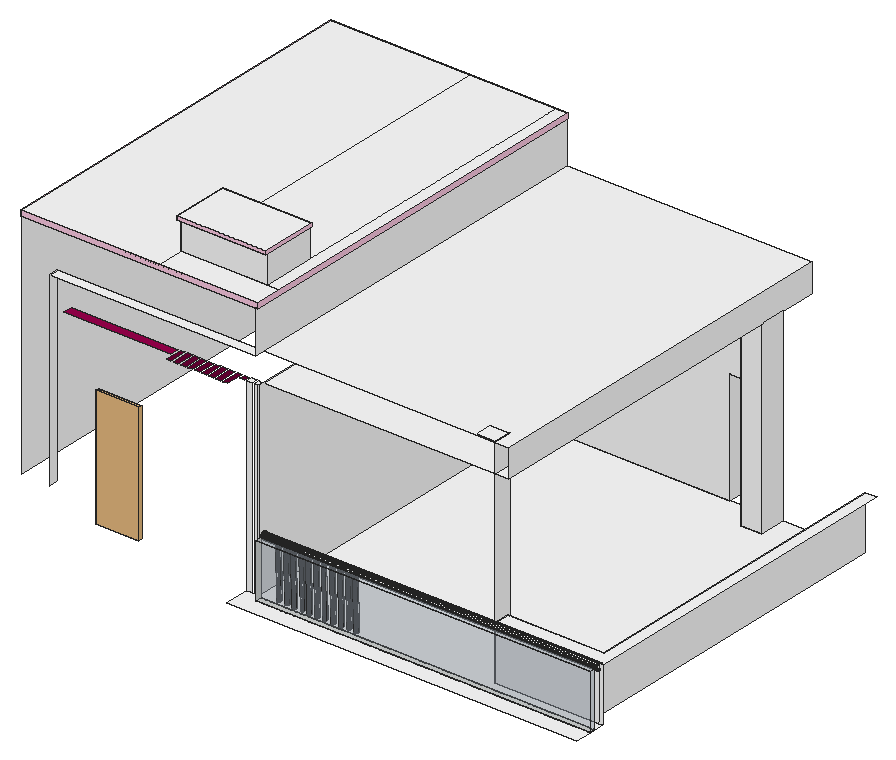
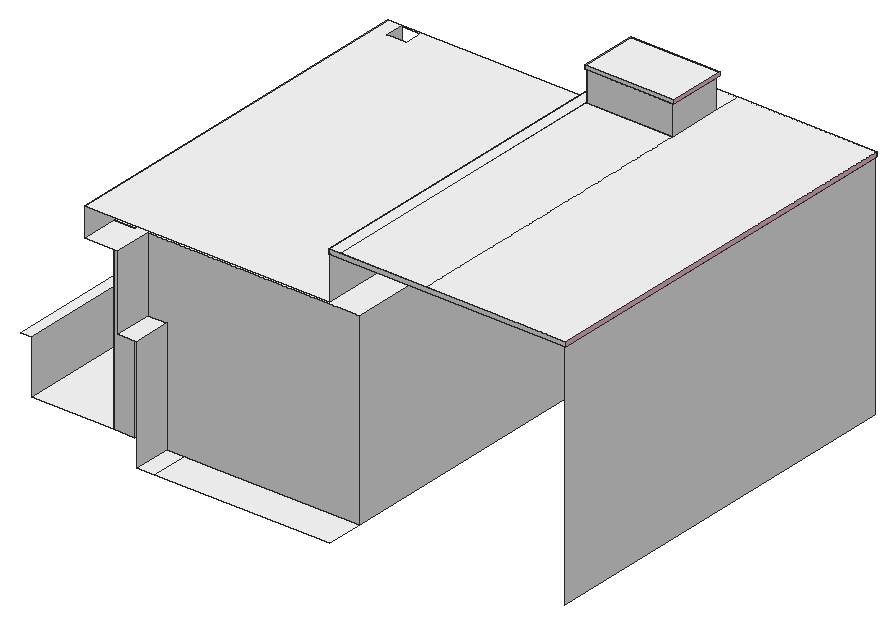
# SketchUp Ruby script. Lengths in inches.
U = 1.inch
M = Sketchup.active_model
def pt(a) = Geom::Point3d.new(a.map { |v| v * U })
def face(e, loops, mat)
  f = e.add_face(loops[0].map { |a| pt(a) })
  loops[1..].each { |l| e.add_face(l.map { |a| pt(a) }).erase! }
  f.material = f.back_material = mat if mat
  f
end
# faces: each face lists its corners as indices into pts; further lists are holes
def faces(e, pts, list, mat = nil) = list.each { |f| face(e, (f[0].is_a?(Array) ? f : [f]).map { |l| l.map { |i| pts[i] } }, mat) }
# xy, xz, yz: faces in a plane at the given z, y or x. An outline is a flat list of corners, or four numbers for a rectangle; further outlines are holes
def ring(l) = l.size == 4 ? [[l[0], l[1]], [l[2], l[1]], [l[2], l[3]], [l[0], l[3]]] : l.each_slice(2).to_a
def flat(e, list, mat, &to3) = list.each { |f| face(e, (f[0].is_a?(Array) ? f : [f]).map { |l| ring(l).map { |u, v| to3.(u, v) } }, mat) }
def xy(e, z, list, mat = nil) = flat(e, list, mat) { |x, y| [x, y, z] }
def xz(e, y, list, mat = nil) = flat(e, list, mat) { |x, z| [x, y, z] }
def yz(e, x, list, mat = nil) = flat(e, list, mat) { |y, z| [x, y, z] }
def lines(e, pts, list) = list.each { |a, b| e.add_line(pt(pts[a]), pt(pts[b])) }
# prism: a flat outline (further loops are holes) pulled along v
def prism(e, loops, v, mat = nil)
  f = face(e, loops, mat); d = Geom::Vector3d.new(v.map { |x| x * U })
  f.pushpull(f.normal.samedirection?(d) ? d.length : -d.length)
end
def box(e, o, s, mat = nil) = prism(e, [[o, [o[0] + s[0], o[1], o[2]], [o[0] + s[0], o[1] + s[1], o[2]], [o[0], o[1] + s[1], o[2]]]], [0, 0, s[2]], mat)
def at(x, y, z, deg = 0) = Geom::Transformation.translation(pt([x, y, z])) * Geom::Transformation.rotation(ORIGIN, Z_AXIS, deg.degrees)
def axes(o, x, y, z) = Geom::Transformation.new([*x, 0, *y, 0, *z, 0, *pt(o).to_a, 1])
def part(name) = M.definitions.add(name)
# library, detail: a bought-in or finely detailed component or shape, given as its bounding box
def library(name, o, s) = part(name).tap { |d| box(d.entities, o, s) }
def detail(e, o, s) = box(e.add_group.entities, o, s)
def put(e, d, t, mat = nil) = e.add_instance(d, t).tap { |i| i.material = mat if mat }
def group(e, t, mat = nil) = e.add_group.tap { |g| g.transformation = t; g.material = mat if mat }.entities
root = M.entities
M.materials.add("Glass_Basic_01").color = [161, 173, 186]
M.materials["Glass_Basic_01"].alpha = 0.25
M.materials.add("L01_Cotton_Candy").color = [255, 204, 229]
M.materials.add("L07_Raspberry_Rush").color = [153, 0, 76]
M.materials.add("L08_Velvet_Rose").color = [102, 0, 51]
M.materials.add("M00_Soft_Cloud").color = [255, 255, 255]
c1 = library("Window 109 023",[-16.24,-1.39,-0.03],[32.48,2.78,89.27])
xy(root,396,[[202.46,150.61,484.6,155.72]])
xy(root,396,[[189,136.44,484.6,136.44,484.6,150.61,202.46,150.61,202.46,155.72,484.6,155.72,484.6,163.42,394.03,163.42,394.03,176.81,475.23,176.81,475.23,451.98,405.98,451.98,405.98,429.82,388.44,429.82,388.44,451.29,199,451.29,199,158.82,198,158.82,198,158.3,189,158.3],[388.44,429.82,405.98,451.98],[199,451.29,346.72,482.39],[346.72,451.29,361.66,482.39]],"M00_Soft_Cloud")
xy(root,437.32,[[198.42,161.79,483.26,161.82]],"M00_Soft_Cloud")
xy(root,441.51,[[394.03,163.42,481.66,164.21],[481.66,163.42,484.6,163.42,484.6,451.98,475.23,451.98,475.23,176.81,394.03,176.81,394.03,164.21,481.66,164.21]],"M00_Soft_Cloud")
xy(root,441.75,[[202.46,150.61,484.6,155.72]],"Glass_Basic_01")
xy(root,491.38,[[361.66,451.29,377.86,482.39]],"M00_Soft_Cloud")
xy(root,554.29,[[37,154.91,127,162.91]],"L07_Raspberry_Rush")
xy(root,554.29,[[129,148,133,162.91],[135,148,139,162.91],[141,148,145,162.91],[147,148,151,162.91],[153,148,157,162.91],
  [159,148,163,162.91],[165,148,169,162.91],[171,148,175,162.91],[177,148,181,162.91],[183,158.3,187,162.91]],"L08_Velvet_Rose")
xy(root,554.29,[[189,158.3,193,162.91],[195,158.3,198,162.91],[198,158.82,199,162.91],[199,162.91,199,451.29,377.86,451.29,377.86,420,405.98,420,405.98,162.91],[377.86,420,377.86,482.39,405.98,482.39,405.98,451.98,388.44,451.98,388.44,429.82,405.98,429.82,405.98,420],
  [388.44,429.82,405.98,451.98]],"M00_Soft_Cloud")
xy(root,578.29,[[25,155.3,199,162.91],[[199,162.91,405.98,482.39],[377.49,163.42,394.03,178.61]]],"M00_Soft_Cloud")
xy(root,614.29,[[0,155.3,1,158.3],[1,155.3,199,482.39],[199,155.3,200,158.3],[0,158.3,1,482.39],[199,158.3,200,482.39]],"M00_Soft_Cloud")
xy(root,618.29,[[0,155.3,117.07,482.39],[117.07,155.3,200,178.22],[117.07,178.22,190.22,223.17],[190.22,178.22,200,482.39],[117.07,223.17,190.22,482.39]],"M00_Soft_Cloud")
xy(root,643.14,[[116.07,175.22,191.22,178.22],[116.07,178.22,117.07,223.17],[190.22,178.22,191.22,223.17]],"L01_Cotton_Candy")
xy(root,643.14,[[117.07,178.22,190.22,223.17]],"M00_Soft_Cloud")
xy(root,646.14,[[116.07,175.22,191.22,223.17]],"M00_Soft_Cloud")
xz(root,150.61,[[202.46,396,484.6,441.75]],"Glass_Basic_01")
xz(root,155.3,[[0,614.29,200,618.29]],"L01_Cotton_Candy")
xz(root,155.72,[[202.46,396,484.6,441.75]],"Glass_Basic_01")
xz(root,158.3,[[189,396,193,554.29],[195,396,198,554.29]],"M00_Soft_Cloud")
xz(root,158.82,[[198,396,199,554.29]],"M00_Soft_Cloud")
xz(root,163.42,[[394.03,396,481.66,441.51],[481.66,396,484.6,441.51]],"M00_Soft_Cloud")
xz(root,175.22,[[116.07,643.14,191.22,646.14]],"L01_Cotton_Candy")
xz(root,176.81,[[394.03,396,398.01,441.51],[398.01,396,475.23,441.51]],"M00_Soft_Cloud")
xz(root,178.22,[[117.07,618.29,190.22,643.14]],"M00_Soft_Cloud")
xz(root,223.17,[[117.07,618.29,190.22,643.14],[116.07,643.14,191.22,646.14]],"M00_Soft_Cloud")
xz(root,429.82,[[388.44,396,405.98,554.29]],"M00_Soft_Cloud")
xz(root,451.29,[[199,396,361.66,396,361.66,491.38,377.86,491.38,377.86,554.29,199,554.29]],"M00_Soft_Cloud")
xz(root,451.98,[[388.44,396,405.98,554.29]],"M00_Soft_Cloud")
xz(root,482.39,[[0,614.29,200,618.29]],"M00_Soft_Cloud")
yz(root,0,[[155.3,614.29,482.39,618.29]],"L01_Cotton_Candy")
yz(root,1,[[155.3,419.15,482.39,614.29]],"M00_Soft_Cloud")
yz(root,25,[[155.3,419.15,162.91,578.29]],"M00_Soft_Cloud")
yz(root,116.07,[[175.22,643.14,223.17,646.14]],"L01_Cotton_Candy")
yz(root,117.07,[[178.22,618.29,223.17,643.14]],"M00_Soft_Cloud")
yz(root,190.22,[[178.22,618.29,223.17,643.14]],"M00_Soft_Cloud")
yz(root,191.22,[[175.22,643.14,223.17,646.14]],"L01_Cotton_Candy")
yz(root,198,[[158.3,396,158.82,554.29]],"M00_Soft_Cloud")
yz(root,199,[[158.82,396,451.29,554.29],[155.3,578.29,482.39,614.29]],"M00_Soft_Cloud")
yz(root,200,[[155.3,614.29,482.39,618.29]],"L01_Cotton_Candy")
yz(root,202.46,[[150.61,396,155.72,441.75]])
yz(root,361.66,[[451.29,396,482.39,491.38]],"M00_Soft_Cloud")
yz(root,377.86,[[451.29,491.38,482.39,554.29]],"M00_Soft_Cloud")
yz(root,388.44,[[429.82,396,451.98,554.29]],"M00_Soft_Cloud")
yz(root,394.03,[[163.42,396,176.81,441.51],[176.81,396,178.61,396,178.61,578.29,163.42,578.29,163.42,441.51,176.81,441.51]],"M00_Soft_Cloud")
yz(root,405.98,[[429.82,396,451.98,554.29],[162.91,554.29,482.39,578.29]],"M00_Soft_Cloud")
yz(root,475.23,[[176.81,396,451.98,441.51]],"M00_Soft_Cloud")
yz(root,484.6,[[150.61,396,155.72,441.75]],"Glass_Basic_01")
p = [[253.49,156.28,440.79],[253.49,157.49,396],[253.91,157.4375,396],[253.91,156.23,440.79],[254.32,157.49,396],[254.32,156.28,440.79],
  [246.48,156.5,440.8],[246.48,157.7,396],[246.87,157.54,396],[246.87,156.34,440.79],[247.28,157.49,396],[247.28,156.28,440.79],
  [247.69,157.54,396],[247.69,156.34,440.79],[248.08,157.7,396],[248.08,156.5,440.8],[253.11,156.44,440.8],[253.11,157.65,396],
  [254.7,157.65,396],[254.7,156.44,440.8],[227.77,156.48,440.79],[227.77,157.6875,396],[228.18,157.63,396],[228.18,156.42,440.79],
  [228.6,157.6875,396],[228.6,156.48,440.79],[252.78,156.69,440.8],[252.78,157.9,396],[255.04,157.9,396],[255.04,156.69,440.8],
  [260.23,156.48,440.79],[260.23,157.68,396],[260.65,157.63,396],[260.65,156.42,440.79],[261.06,157.68,396],[261.06,156.48,440.79],
  [227.38,156.64,440.8],[227.38,157.85,396],[228.98,157.85,396],[228.98,156.64,440.8],[246.15,156.75,440.8],[246.15,157.96,396],
  [248.41,157.96,396],[248.41,156.75,440.8],[259.85,156.64,440.8],[259.85,157.84,396],[261.44,157.84,396],[261.44,156.64,440.8],
  [267.02,156.68,440.8],[267.02,157.89,396],[267.4,157.73,396],[267.4,156.52,440.79],[267.82,157.68,396],[267.82,156.47,440.79],
  [268.23,157.73,396],[268.23,156.52,440.79],[268.62,157.89,396],[268.62,156.68,440.8],[227.05,156.89,440.8],[227.05,158.1,396],
  [229.3125,158.1,396],[229.3125,156.89,440.8],[259.52,156.89,440.8],[259.52,158.1,396],[261.78,158.1,396],[261.78,156.89,440.8],
  [245.9,157.08,440.8125],[245.9,158.29,396],[248.66,158.29,396],[248.66,157.08,440.8125],[252.52,157.03,440.8125],[252.52,158.23,396],
  [255.29,158.23,396],[255.29,157.03,440.8125],[266.6875,156.94,440.8],[266.6875,158.14,396],[268.95,158.14,396],[268.95,156.94,440.8],
  [279.15,156.99,440.8],[279.15,158.2,396],[279.53,158.04,396],[279.53,156.83,440.79],[279.95,157.99,396],[279.95,156.78,440.79],
  [280.36,158.04,396],[280.36,156.83,440.79],[280.74,158.2,396],[280.74,156.99,440.8],[226.8,157.22,440.8125],[226.8,158.43,396],
  [229.57,158.43,396],[229.57,157.22,440.8125],[239.74,157.07,440.8],[239.74,158.28,396],[240.125,158.12,396],[240.125,156.91,440.79],
  [240.54,158.0625,396],[240.54,156.85,440.79],[240.95,158.12,396],[240.95,156.91,440.79],[241.34,158.28,396],[241.34,157.07,440.8],
  [259.26,157.22,440.8125],[259.26,158.43,396],[262.03,158.43,396],[262.03,157.22,440.8125],[266.43,157.27,440.8125],[266.43,158.48,396],
  [269.2,158.48,396],[269.2,157.27,440.8125],[252.36,157.41,440.82],[252.36,158.62,396],[255.45,158.62,396],[255.45,157.41,440.82],
  [278.82,157.24,440.8],[278.82,158.45,396],[281.08,158.45,396],[281.08,157.24,440.8],[239.41,157.32,440.8],[239.41,158.53,396],
  [241.67,158.53,396],[241.67,157.32,440.8],[245.74,157.47,440.82],[245.74,158.67,396],[248.82,158.67,396],[248.82,157.47,440.82],
  [226.64,157.61,440.82],[226.64,158.82,396],[229.73,158.82,396],[229.73,157.61,440.82],[259.1,157.61,440.82],[259.1,158.81,396],
  [262.1875,158.81,396],[262.1875,157.61,440.82],[278.5625,157.58,440.8125],[278.5625,158.78,396],[281.33,158.78,396],[281.33,157.58,440.8125],
  [234,157.37,440.79],[234,158.58,396],[234.42,158.53,396],[234.42,157.32,440.79],[234.83,158.58,396],[234.83,157.37,440.79],
  [239.15,157.65,440.8125],[239.15,158.86,396],[241.92,158.86,396],[241.92,157.65,440.8125],[266.27,157.65,440.82],[266.27,158.86,396],
  [269.36,158.86,396],[269.36,157.65,440.82],[233.62,157.53,440.8],[233.62,158.74,396],[235.21,158.74,396],[235.21,157.53,440.8],
  [252.31,157.82,440.83],[252.31,159.03,396],[255.5,159.03,396],[255.5,157.82,440.83],[272.5625,157.59,440.8],[272.5625,158.8,396],
  [272.95,158.64,396],[272.95,157.43,440.79],[273.36,158.59,396],[273.36,157.38,440.79],[273.77,158.64,396],[273.77,157.43,440.79],
  [274.16,158.8,396],[274.16,157.59,440.8],[233.29,157.78,440.8],[233.29,158.99,396],[235.55,158.99,396],[235.55,157.78,440.8],
  [245.68,157.88,440.83],[245.68,159.09,396],[248.88,159.09,396],[248.88,157.88,440.83],[213.7,157.7,440.79],[213.7,158.91,396],
  [214.11,158.86,396],[214.11,157.65,440.79],[214.52,158.91,396],[214.52,157.7,440.79],[226.58,158.02,440.83],[226.58,159.23,396],
  [229.78,159.23,396],[229.78,158.02,440.83],[259.05,158.02,440.83],[259.05,159.23,396],[262.24,159.23,396],[262.24,158.02,440.83],
  [272.23,157.85,440.8],[272.23,159.06,396],[274.49,159.06,396],[274.49,157.85,440.8],[278.4,157.96,440.82],[278.4,159.17,396],
  [281.49,159.17,396],[281.49,157.96,440.82],[213.3125,157.86,440.8],[213.3125,159.07,396],[214.91,159.07,396],[214.91,157.86,440.8],
  [220.625,157.78,440.79],[220.625,158.99,396],[221.04,158.9375,396],[221.04,157.73,440.79],[221.45,158.99,396],[221.45,157.78,440.79],
  [238.99,158.04,440.82],[238.99,159.25,396],[242.08,159.25,396],[242.08,158.04,440.82],[266.22,158.06,440.83],[266.22,159.27,396],
  [269.41,159.27,396],[269.41,158.06,440.83],[220.24,157.94,440.8],[220.24,159.15,396],[221.84,159.15,396],[221.84,157.94,440.8],
  [233.03,158.12,440.8125],[233.03,159.32,396],[235.8,159.32,396],[235.8,158.12,440.8125],[252.36,159.45,396.01],[252.36,158.24,440.84],
  [255.45,159.45,396.01],[255.45,158.24,440.84],[271.98,158.18,440.8125],[271.98,159.39,396],[274.74,159.39,396],[274.74,158.18,440.8125],
  [212.98,158.11,440.8],[212.98,159.32,396],[215.24,159.32,396],[215.24,158.11,440.8],[219.91,158.2,440.8],[219.91,159.4,396],
  [222.17,159.4,396],[222.17,158.2,440.8],[245.74,159.5,396.01],[245.74,158.29,440.84],[248.82,159.5,396.01],[248.82,158.29,440.84],
  [226.64,159.64,396.01],[226.64,158.43,440.84],[229.73,159.64,396.01],[229.73,158.43,440.84],[238.94,158.45,440.83],[238.94,159.66,396],
  [242.14,159.66,396],[242.14,158.45,440.83],[259.1,159.64,396.01],[259.1,158.43,440.84],[262.1875,159.64,396.01],[262.1875,158.43,440.84],
  [278.35,158.375,440.83],[278.35,159.58,396],[281.54,159.58,396],[281.54,158.375,440.83],[212.73,158.45,440.8125],[212.73,159.65,396],
  [215.49,159.65,396],[215.49,158.45,440.8125],[232.87,158.5,440.82],[232.87,159.71,396],[235.96,159.71,396],[235.96,158.5,440.82],
  [266.27,159.6875,396.01],[266.27,158.48,440.84],[269.36,159.6875,396.01],[269.36,158.48,440.84],[219.65,158.53,440.8125],[219.65,159.74,396],
  [222.42,159.74,396],[222.42,158.53,440.8125],[252.52,159.83,396.02],[252.52,158.62,440.85],[255.29,159.83,396.02],[255.29,158.62,440.85],
  [271.82,158.5625,440.82],[271.82,159.77,396],[274.9,159.77,396],[274.9,158.5625,440.82],[245.9,159.89,396.02],[245.9,158.68,440.85],
  [248.66,159.89,396.02],[248.66,158.68,440.85],[212.57,158.83,440.82],[212.57,160.04,396],[215.65,160.04,396],[215.65,158.83,440.82],
  [226.8,160.03,396.02],[226.8,158.82,440.85],[229.57,160.03,396.02],[229.57,158.82,440.85],[259.26,160.03,396.02],[259.26,158.82,440.85],
  [262.03,160.03,396.02],[262.03,158.82,440.85],[278.4,160,396.01],[278.4,158.79,440.84],[281.49,160,396.01],[281.49,158.79,440.84],
  [219.49,158.91,440.82],[219.49,160.12,396],[222.58,160.12,396],[222.58,158.91,440.82],[232.82,158.91,440.83],[232.82,160.125,396],
  [236.01,160.125,396],[236.01,158.91,440.83],[238.99,160.07,396.01],[238.99,158.86,440.84],[242.08,160.07,396.01],[242.08,158.86,440.84],
  [266.43,160.07,396.02],[266.43,158.86,440.85],[269.2,160.07,396.02],[269.2,158.86,440.85],[252.78,160.16,396.03],[252.78,158.95,440.86],
  [255.04,160.16,396.03],[255.04,158.95,440.86],[271.76,158.98,440.83],[271.76,160.1875,396],[274.96,160.1875,396],[274.96,158.98,440.83],
  [246.15,160.22,396.03],[246.15,159.01,440.86],[248.41,160.22,396.03],[248.41,159.01,440.86],[212.51,159.24,440.83],[212.51,160.45,396],
  [215.71,160.45,396],[215.71,159.24,440.83],[227.05,160.36,396.03],[227.05,159.15,440.86],[229.3125,160.36,396.03],[229.3125,159.15,440.86],
  [259.52,160.36,396.03],[259.52,159.15,440.86],[261.78,160.36,396.03],[261.78,159.15,440.86],[278.5625,160.38,396.02],[278.5625,159.17,440.85],
  [281.33,160.38,396.02],[281.33,159.17,440.85],[219.44,159.32,440.83],[219.44,160.53,396],[222.64,160.53,396],[222.64,159.32,440.83],
  [232.87,160.54,396.01],[232.84,159.1,440.84],[232.87,159.33,440.84],[235.96,160.54,396.01],[235.96,159.33,440.84],[235.99,159.1,440.84],
  [239.15,160.46,396.02],[239.15,159.25,440.85],[241.92,160.46,396.02],[241.92,159.25,440.85],[266.6875,160.4,396.03],[266.6875,159.19,440.86],
  [268.95,160.4,396.03],[268.95,159.19,440.86],[246.48,160.47,396.04],[246.48,159.26,440.87],[248.08,160.47,396.04],[248.08,159.26,440.87],
  [253.11,160.42,396.04],[253.11,159.21,440.87],[254.7,160.42,396.04],[254.7,159.21,440.87],[271.82,160.6,396.01],[271.82,159.39,440.84],
  [274.9,160.6,396.01],[274.9,159.39,440.84],[259.85,160.61,396.04],[259.85,159.4,440.87],[261.44,160.61,396.04],[261.44,159.4,440.87],
  [212.57,160.87,396.01],[212.57,159.66,440.84],[215.65,160.87,396.01],[215.65,159.66,440.84],[227.38,160.61,396.04],[227.38,159.4,440.87],
  [228.98,160.61,396.04],[228.98,159.4,440.87],[239.41,160.79,396.03],[239.41,159.58,440.86],[241.67,160.79,396.03],[241.67,159.58,440.86],
  [253.49,160.58,396.04],[253.49,159.37,440.875],[254.32,160.58,396.04],[254.32,159.37,440.875],[267.02,160.66,396.04],[267.02,159.45,440.87],
  [268.62,160.66,396.04],[268.62,159.45,440.87],[278.82,160.71,396.03],[278.82,159.5,440.86],[281.08,160.71,396.03],[281.08,159.5,440.86],
  [219.49,160.95,396.01],[219.49,159.74,440.84],[222.58,160.95,396.01],[222.58,159.74,440.84],[233.03,160.92,396.02],[233.03,159.71,440.85],
  [235.8,160.92,396.02],[235.8,159.71,440.85],[246.87,160.63,396.04],[246.87,159.42,440.875],[247.69,160.63,396.04],[247.69,159.42,440.875],
  [227.77,160.77,396.04],[227.77,159.5625,440.875],[228.6,160.77,396.04],[228.6,159.5625,440.875],[247.28,160.69,396.04],[247.28,159.48,440.875],
  [253.91,160.63,396.04],[253.91,159.42,440.875],[260.23,160.77,396.04],[260.23,159.5625,440.875],[261.06,160.77,396.04],[261.06,159.5625,440.875],
  [267.4,160.82,396.04],[267.4,159.61,440.875],[268.23,160.82,396.04],[268.23,159.61,440.875],[271.98,160.99,396.02],[271.98,159.78,440.85],
  [274.74,160.99,396.02],[274.74,159.78,440.85],[279.15,160.97,396.04],[279.15,159.76,440.87],[280.74,160.97,396.04],[280.74,159.76,440.87],
  [228.18,160.83,396.04],[228.18,159.62,440.875],[239.74,161.04,396.04],[239.74,159.83,440.87],[241.34,161.04,396.04],[241.34,159.83,440.87],
  [260.65,160.83,396.04],[260.65,159.62,440.875],[267.82,160.87,396.04],[267.82,159.66,440.875],[212.73,161.25,396.02],[212.73,160.04,440.85],
  [215.49,161.25,396.02],[215.49,160.04,440.85],[219.65,161.33,396.02],[219.65,160.125,440.85],[222.42,161.33,396.02],[222.42,160.125,440.85],
  [233.29,161.25,396.03],[233.29,160.04,440.86],[235.55,161.25,396.03],[235.55,160.04,440.86],[240.125,161.2,396.04],[240.125,159.99,440.875],
  [240.95,161.2,396.04],[240.95,159.99,440.875],[272.23,161.32,396.03],[272.23,160.11,440.86],[274.49,161.32,396.03],[274.49,160.11,440.86],
  [279.53,161.125,396.04],[279.53,159.92,440.875],[280.36,161.125,396.04],[280.36,159.92,440.875],[279.95,161.18,396.04],[279.95,159.97,440.875],
  [212.98,161.58,396.03],[212.98,160.37,440.86],[215.24,161.58,396.03],[215.24,160.37,440.86],[233.62,161.51,396.04],[233.62,160.3,440.87],
  [235.21,161.51,396.04],[235.21,160.3,440.87],[240.54,161.26,396.04],[240.54,160.05,440.875],[219.91,161.66,396.03],[219.91,160.45,440.86],
  [222.17,161.66,396.03],[222.17,160.45,440.86],[272.5625,161.57,396.04],[272.5625,160.36,440.87],[274.16,161.57,396.04],[274.16,160.36,440.87],
  [234,161.67,396.04],[234,160.46,440.875],[234.83,161.67,396.04],[234.83,160.46,440.875],[213.3125,161.84,396.04],[213.3125,160.625,440.87],
  [214.91,161.84,396.04],[214.91,160.625,440.87],[272.95,161.73,396.04],[272.95,160.52,440.875],[273.77,161.73,396.04],[273.77,160.52,440.875],
  [220.24,161.92,396.04],[220.24,160.71,440.87],[221.84,161.92,396.04],[221.84,160.71,440.87],[234.42,161.72,396.04],[234.42,160.51,440.875],
  [273.36,161.78,396.04],[273.36,160.57,440.875],[213.7,162,396.04],[213.7,160.79,440.875],[214.52,162,396.04],[214.52,160.79,440.875],
  [220.625,162.08,396.04],[220.625,160.87,440.875],[221.45,162.08,396.04],[221.45,160.87,440.875],[214.11,162.05,396.04],[214.11,160.84,440.875],
  [221.04,162.13,396.04],[221.04,160.92,440.875],[483.26,161.07,437.42],[198.42,161.07,437.42],[198.42,161.79,437.32],[483.26,161.79,437.32],
  [214.37,161.82,437.32],[211.17,161.82,437.32],[198.42,161.82,437.32],[198.42,162.52,437.42],[483.26,162.52,437.42],[483.26,161.82,437.32],
  [269.19,161.82,437.32],[265.99,161.82,437.32],[261.87,161.82,437.32],[258.67,161.82,437.32],[254.93,161.82,437.32],[251.74,161.82,437.32],
  [248.04,161.82,437.32],[244.84,161.82,437.32],[241.38,161.82,437.32],[238.1875,161.82,437.32],[235.53,161.82,437.32],[232.34,161.82,437.32],
  [228.79,161.82,437.32],[225.6,161.82,437.32],[221.49,161.82,437.32],[218.29,161.82,437.32],[483.26,160.4,437.69],[198.42,160.4,437.69],
  [198.42,163.19,437.69],[483.26,163.19,437.69],[483.26,159.82,438.14],[198.42,159.82,438.14],[198.42,163.77,438.14],[483.26,163.77,438.14],
  [483.26,159.375,438.72],[198.42,159.375,438.72],[198.42,164.21,438.72],[483.26,164.21,438.72],[483.26,159.1,439.39],[198.42,159.1,439.39],
  [198.42,164.49,439.39],[483.26,164.49,439.39],[483.26,159,440.11],[198.42,159,440.11],[198.42,164.59,440.11],[483.26,164.59,440.11],
  [198.42,159.1,440.84],[483.26,159.1,440.84],[198.42,164.49,440.84],[483.26,164.49,440.84],[483.26,159.375,441.51],[198.42,159.375,441.51],
  [198.42,164.21,441.51],[394.03,164.21,441.51],[481.66,164.21,441.51],[483.26,164.21,441.51],[483.26,159.82,442.09],[198.42,159.82,442.09],
  [198.42,163.77,442.09],[483.26,163.77,442.09],[483.26,160.4,442.53],[198.42,160.4,442.53],[198.42,163.19,442.53],[483.26,163.19,442.53],
  [483.26,161.07,442.8125],[198.42,161.07,442.8125],[198.42,162.52,442.8125],[483.26,162.52,442.8125],[483.26,161.79,442.91],[198.42,161.79,442.91]]
faces(root,p,[[0,1,2,3],[3,2,4,5],[6,7,8,9],[9,8,10,11],[11,10,12,13],[13,12,14,15],[16,17,1,0],[5,4,18,19],
  [20,21,22,23],[23,22,24,25],[26,27,17,16],[19,18,28,29],[30,31,32,33],[33,32,34,35],[36,37,21,20],[25,24,38,39],
  [40,41,7,6],[15,14,42,43],[44,45,31,30],[35,34,46,47],[48,49,50,51],[51,50,52,53],[53,52,54,55],[55,54,56,57],
  [58,59,37,36],[39,38,60,61],[62,63,45,44],[47,46,64,65],[66,67,41,40],[43,42,68,69],[70,71,27,26],[29,28,72,73],
  [74,75,49,48],[57,56,76,77],[78,79,80,81],[81,80,82,83],[83,82,84,85],[85,84,86,87],[88,89,59,58],[61,60,90,91],
  [92,93,94,95],[95,94,96,97],[97,96,98,99],[99,98,100,101],[102,103,63,62],[65,64,104,105],[106,107,75,74],[77,76,108,109],
  [110,111,71,70],[73,72,112,113],[114,115,79,78],[87,86,116,117],[118,119,93,92],[101,100,120,121],[122,123,67,66],[69,68,124,125],
  [126,127,89,88],[91,90,128,129],[130,131,103,102],[105,104,132,133],[134,135,115,114],[117,116,136,137],[138,139,140,141],[141,140,142,143],
  [144,145,119,118],[121,120,146,147],[148,149,107,106],[109,108,150,151],[152,153,139,138],[143,142,154,155],[156,157,111,110],[113,112,158,159],
  [160,161,162,163],[163,162,164,165],[165,164,166,167],[167,166,168,169],[170,171,153,152],[155,154,172,173],[174,175,123,122],[125,124,176,177],
  [178,179,180,181],[181,180,182,183],[184,185,127,126],[129,128,186,187],[188,189,131,130],[133,132,190,191],[192,193,161,160],[169,168,194,195],
  [196,197,135,134],[137,136,198,199],[200,201,179,178],[183,182,202,203],[204,205,206,207],[207,206,208,209],[210,211,145,144],[147,146,212,213],
  [214,215,149,148],[151,150,216,217],[218,219,205,204],[209,208,220,221],[222,223,171,170],[173,172,224,225],[226,157,156,227],[158,228,229,159],
  [230,231,193,192],[195,194,232,233],[234,235,201,200],[203,202,236,237],[238,239,219,218],[221,220,240,241],[242,175,174,243],[176,244,245,177],
  [246,185,184,247],[186,248,249,187],[250,251,211,210],[213,212,252,253],[254,189,188,255],[190,256,257,191],[258,259,197,196],[199,198,260,261],
  [262,263,235,234],[237,236,264,265],[266,267,223,222],[225,224,268,269],[270,215,214,271],[216,272,273,217],[274,275,239,238],[241,240,276,277],
  [278,226,227,279],[228,280,281,229],[282,283,231,230],[233,232,284,285],[286,242,243,287],[244,288,289,245],[290,291,263,262],[265,264,292,293],
  [294,246,247,295],[248,296,297,249],[298,254,255,299],[256,300,301,257],[302,259,258,303],[260,304,305,261],[306,307,275,274],[277,276,308,309],
  [310,311,267,266],[269,268,312,313],[314,251,250,315],[252,316,317,253],[318,270,271,319],[272,320,321,273],[322,278,279,323],[280,324,325,281],
  [326,327,283,282],[285,284,328,329],[330,286,287,331],[288,332,333,289],[334,335,291,290],[293,292,336,337],[338,294,295,339],[296,340,341,297],
  [342,298,299,343],[300,344,345,301],[346,302,303,347],[304,348,349,305],[350,351,307,306],[309,308,352,353],[354,311,310,355,356],[312,357,358,359,313],
  [360,314,315,361],[316,362,363,317],[364,318,319,365],[320,366,367,321],[368,330,331,369],[332,370,371,333],[372,322,323,373],[324,374,375,325],
  [376,327,326,377],[328,378,379,329],[380,342,343,381],[344,382,383,345],[384,335,334,385],[336,386,387,337],[388,338,339,389],[340,390,391,341],
  [392,360,361,393],[362,394,395,363],[396,372,373,397],[374,398,399,375],[400,364,365,401],[366,402,403,367],[404,346,347,405],[348,406,407,349],
  [408,351,350,409],[352,410,411,353],[412,354,356,413],[357,414,415,358],[416,368,369,417],[370,418,419,371],[420,388,389,421],[390,422,423,391],
  [424,416,417,425],[418,424,425,419],[426,396,397,427],[398,426,427,399],[428,380,381,429],[382,430,431,383],[432,400,401,433],[402,434,435,403],
  [436,376,377,437],[378,438,439,379],[440,404,405,441],[406,442,443,407],[444,420,421,445],[422,444,445,423],[446,392,393,447],[394,448,449,395],
  [450,428,429,451],[430,450,451,431],[452,432,433,453],[434,452,453,435],[454,384,385,455],[386,456,457,387],[458,408,409,459],[410,460,461,411],
  [462,412,413,463],[414,464,465,415],[466,446,447,467],[448,468,469,449],[470,436,437,471],[438,472,473,439],[474,440,441,475],[442,476,477,443],
  [478,474,475,479],[476,478,479,477],[480,454,455,481],[456,482,483,457],[484,462,463,485],[464,486,487,465],[488,466,467,489],[468,488,489,469],
  [490,458,459,491],[460,492,493,461],[494,470,471,495],[472,496,497,473],[498,484,485,499],[486,500,501,487],[502,480,481,503],[482,504,505,483],
  [506,494,495,507],[496,508,509,497],[510,490,491,511],[492,512,513,493],[514,498,499,515],[500,514,515,501],[516,506,507,517],[508,516,517,509],
  [518,502,503,519],[504,520,521,505],[522,510,511,523],[512,524,525,513],[526,518,519,527],[520,526,527,521],[528,522,523,529],[524,528,529,525],
  [530,531,532,533],[534,535,536,537,538,539,540,541,542,543,544,545,546,547,548,549,550,551,552,553,554,555],[556,557,531,530],[538,537,558,559],[560,561,557,556],[559,558,562,563],[564,565,561,560],[563,562,566,567],
  [568,569,565,564],[567,566,570,571],[572,573,569,568],[571,570,574,575],[355,576,573,572,577,359],[575,574,578,579],[580,581,576,355,359,577],[579,578,582,583,584,585],
  [586,587,581,580],[583,582,588,589,585,584],[590,591,587,586],[589,588,592,593],[594,595,591,590],[593,592,596,597],[598,599,595,594],[597,596,599,598]],"M00_Soft_Cloud")
put(root,c1,axes([82.15,156.34,404.03],[1.12885,0,0],[0,1.03378,0],[0,0,1.12919]))
